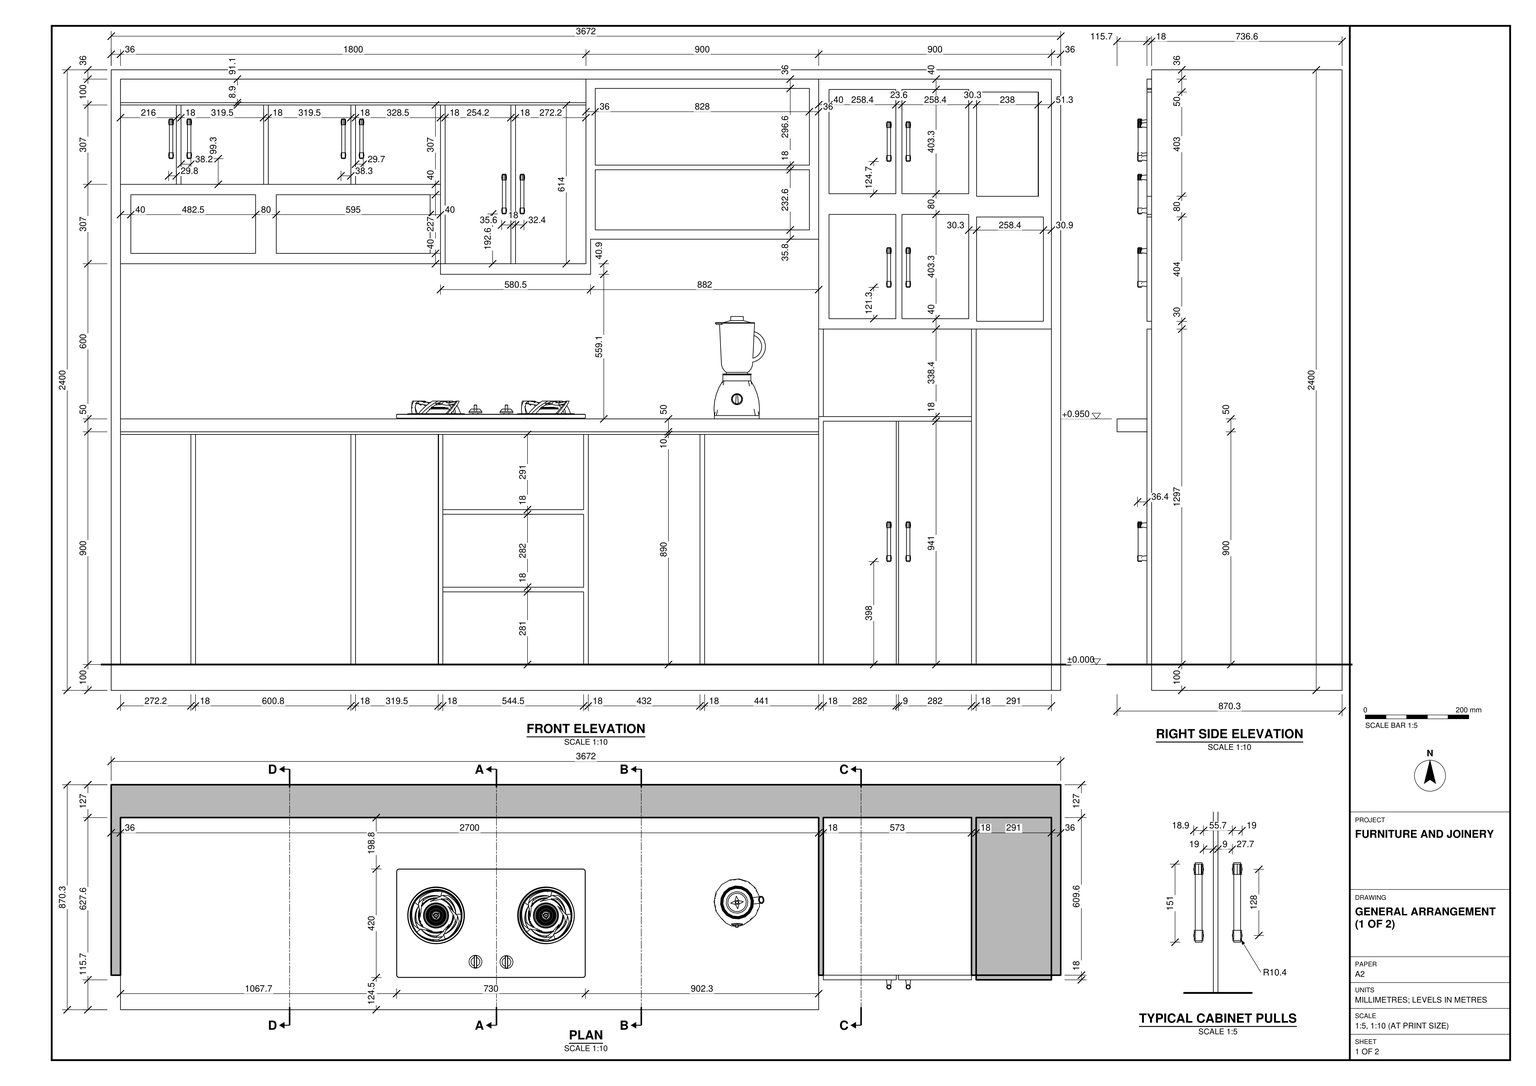
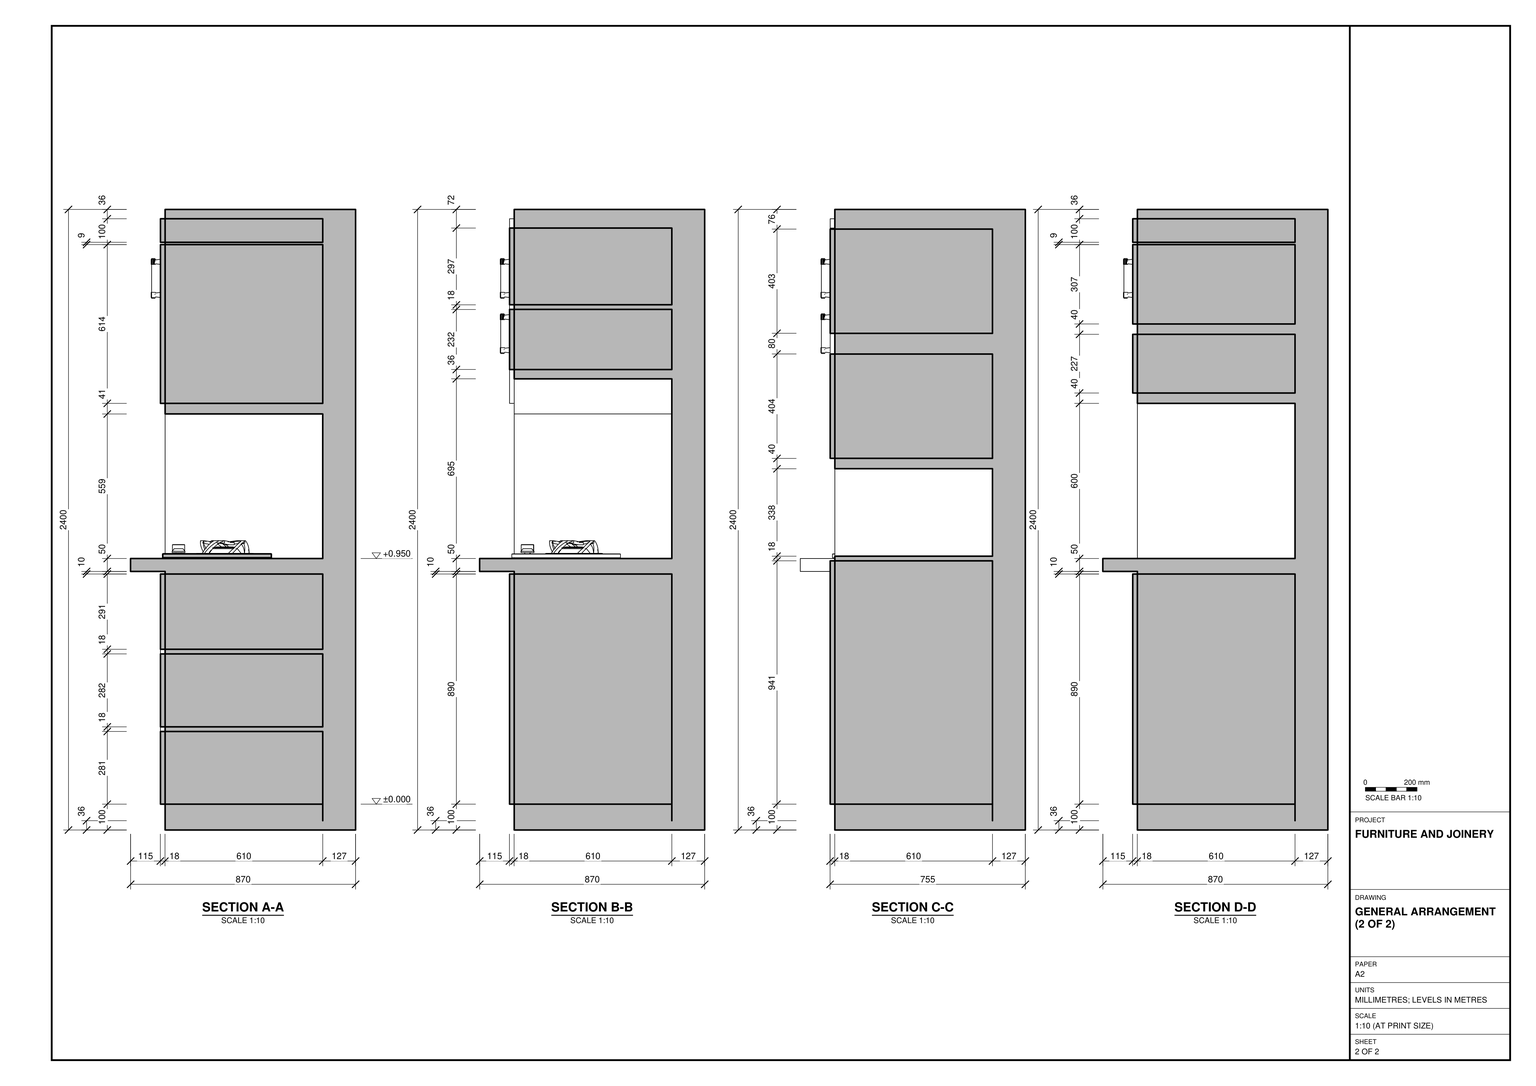
Build the fitted kitchen joinery in SketchUp from task_files/diagram_01.pdf. Work in millimetres. The complete unit is 3672 mm wide, 870.3 mm deep and 2400 mm high. Use the floor line marked ±0.000 as the 0 mm datum. The base of the surround is 100 mm below this line, and the worktop surface is 950 mm above it.

Use the plan and front elevation to lay out the backing, end panels, base cabinets and upper cabinets. Run the worktop across the left-hand base cabinets and stop it at the tall storage section on the right. Use the sections on the second sheet to set the panel thicknesses, shelf heights and projection of the worktop beyond the cabinet fronts. Match the stacked compartments below the cooktop, the changing heights of the upper cupboards and the open shelf bay beside them. Fit vertical pulls to the doors indicated in the elevation. Place the cooktop and countertop mixer in their plan positions.

Make the surround, worktop and each distinct cabinet assembly separate groups or components, and use components for repeated parts such as pulls. Appliances, decor and loose items may be any suitable library components. Save one SketchUp model as output_files/fitted_kitchen_cabinet_run_with_a_projecting_worktop.skp.

# SketchUp Ruby script. Lengths in millimetres.
U = 1.mm
M = Sketchup.active_model
def pt(a) = Geom::Point3d.new(a.map { |v| v * U })
def face(e, loops, mat)
  f = e.add_face(loops[0].map { |a| pt(a) })
  loops[1..].each { |l| e.add_face(l.map { |a| pt(a) }).erase! }
  f.material = f.back_material = mat if mat
  f
end
# faces: each face lists its corners as indices into pts; further lists are holes
def faces(e, pts, list, mat = nil) = list.each { |f| face(e, (f[0].is_a?(Array) ? f : [f]).map { |l| l.map { |i| pts[i] } }, mat) }
# xy, xz, yz: faces in a plane at the given z, y or x. An outline is a flat list of corners, or four numbers for a rectangle; further outlines are holes
def ring(l) = l.size == 4 ? [[l[0], l[1]], [l[2], l[1]], [l[2], l[3]], [l[0], l[3]]] : l.each_slice(2).to_a
def flat(e, list, mat, &to3) = list.each { |f| face(e, (f[0].is_a?(Array) ? f : [f]).map { |l| ring(l).map { |u, v| to3.(u, v) } }, mat) }
def xy(e, z, list, mat = nil) = flat(e, list, mat) { |x, y| [x, y, z] }
def xz(e, y, list, mat = nil) = flat(e, list, mat) { |x, z| [x, y, z] }
def yz(e, x, list, mat = nil) = flat(e, list, mat) { |y, z| [x, y, z] }
def lines(e, pts, list) = list.each { |a, b| e.add_line(pt(pts[a]), pt(pts[b])) }
# prism: a flat outline (further loops are holes) pulled along v
def prism(e, loops, v, mat = nil)
  f = face(e, loops, mat); d = Geom::Vector3d.new(v.map { |x| x * U })
  f.pushpull(f.normal.samedirection?(d) ? d.length : -d.length)
end
def box(e, o, s, mat = nil) = prism(e, [[o, [o[0] + s[0], o[1], o[2]], [o[0] + s[0], o[1] + s[1], o[2]], [o[0], o[1] + s[1], o[2]]]], [0, 0, s[2]], mat)
def at(x, y, z, deg = 0) = Geom::Transformation.translation(pt([x, y, z])) * Geom::Transformation.rotation(ORIGIN, Z_AXIS, deg.degrees)
def axes(o, x, y, z) = Geom::Transformation.new([*x, 0, *y, 0, *z, 0, *pt(o).to_a, 1])
def part(name) = M.definitions.add(name)
# library, detail: a bought-in or finely detailed component or shape, given as its bounding box
def library(name, o, s) = part(name).tap { |d| box(d.entities, o, s) }
def detail(e, o, s) = box(e.add_group.entities, o, s)
def put(e, d, t, mat = nil) = e.add_instance(d, t).tap { |i| i.material = mat if mat }
def group(e, t, mat = nil) = e.add_group.tap { |g| g.transformation = t; g.material = mat if mat }.entities
root = M.entities
M.materials.add("0257 AP 9616 Wisteria Lane-N").color = [173, 152, 201]
M.materials.add("0466 AP 9679 Little Andaman-N").color = [89, 168, 184]
M.materials.add("0522 AP 7474 SAPPHIRE ICE").color = [176, 207, 204]
M.materials.add("CLC2-PC-Blanc INTER").color = [249, 249, 249]
M.materials.add("[Color M00]").color = [255, 255, 255]
M.materials.add("[Color M09]").color = [0, 0, 0]
M.materials.add("[Translucent Glass Blue]").color = [100, 149, 237]
M.materials["[Translucent Glass Blue]"].alpha = 0.5
M.materials.add("[Wood Floor]").color = [155, 105, 61]
c1 = library("2-PRODUITS CUISINE CLC2",[-33.7,-33.7,0],[67.4,67.4,274.4])
c2 = library("1-PRODUITS CUISINE CLC2\#1",[-28.3,-28.3,0],[56.6,56.6,273])
c3 = library("GasStove_Black",[0,0,0],[730,420,69])
c4 = part("CLC2-Ele02")
prism(c4.entities,[[[-0.2,-8.1,4],[-0.2,-8.3,0.4],[-0.2,-8.7,-3.2],[-0.2,-9.2,-6.8],[-0.2,-9.9,-10.3],[-0.2,-10.8,-13.9],[-0.2,-11.8,-17.3],[-0.2,-13,-20.8],[-0.2,-5.2,-21.4],[-0.2,-1.7,21.4],[-0.2,-9.5,22.1],[-0.2,-8.9,18.5],[-0.2,-8.5,14.9],[-0.2,-8.2,11.3],[-0.2,-8.1,7.7]]],[-21.2,0,0],"[Color M00]")
xy(c4.entities,-40,[[-36.6,-4.9,36.6,0]],"CLC2-PC-Blanc INTER")
xy(c4.entities,-38,[[-34.9,-2.9,34.9,0]],"CLC2-PC-Blanc INTER")
xy(c4.entities,-22,[[-21.5,-7.3,21.5,-2.9]],"CLC2-PC-Blanc INTER")
xy(c4.entities,22,[[-21.5,-7.3,21.5,-2.9]],"CLC2-PC-Blanc INTER")
xy(c4.entities,38,[[-34.9,-2.9,34.9,0]],"CLC2-PC-Blanc INTER")
xy(c4.entities,40,[[-36.6,-4.9,36.6,0]],"CLC2-PC-Blanc INTER")
xz(c4.entities,-8.1,[[0.2,4,21.4,7.7]],"[Color M00]")
xz(c4.entities,-2.9,[[[-34.9,-38,-35.7,-33.1,-36.5,-26.5,-37.2,-19.9,-37.7,-13.3,-38,-6.6,-38,6.6,-37.7,13.3,-37.2,19.9,-36.5,26.5,-35.7,33.1,-34.9,38,34.9,38,35.7,33.1,36.5,26.5,37.2,19.9,37.7,13.3,38,6.6,38,-6.6,37.7,-13.3,37.2,-19.9,36.5,-26.5,35.7,-33.1,34.9,-38],[-21.5,-22,21.5,22]]],"CLC2-PC-Blanc INTER")
xz(c4.entities,0,[[-36.6,-40,-37.6,-33.4,-38.5,-26.7,-39.1,-20.1,-39.6,-13.4,-39.9,-6.7,-40,0,-39.9,6.7,-39.6,13.4,-39.1,20.1,-38.5,26.7,-37.6,33.4,-36.6,40,0,40,0,38,-34.9,38,-35.7,33.1,-36.5,26.5,-37.2,19.9,-37.7,13.3,-38,6.6,-38,-6.6,-37.7,-13.3,-37.2,-19.9,-36.5,-26.5,-35.7,-33.1,-34.9,-38,0,-38,0,-40],[0,-40,0,-38,34.9,-38,35.7,-33.1,36.5,-26.5,37.2,-19.9,37.7,-13.3,38,-6.6,38,6.6,37.7,13.3,37.2,19.9,36.5,26.5,35.7,33.1,34.9,38,0,38,0,40,36.6,40,37.6,33.4,38.5,26.7,39.1,20.1,39.6,13.4,39.9,6.7,40,0,39.9,-6.7,39.6,-13.4,39.1,-20.1,38.5,-26.7,37.6,-33.4,36.6,-40]],"CLC2-PC-Blanc INTER")
yz(c4.entities,-38,[[-2.9,-6.6,0,0],[-2.9,0,0,6.6]],"CLC2-PC-Blanc INTER")
yz(c4.entities,-21.5,[[-7.3,-22,-2.9,-22,-2.9,22,-7.3,22,-7.5,20.1,-8,13.4,-8.2,6.7,-8.3,0,-8.2,-6.7,-8,-13.4,-7.5,-20.1]],"CLC2-PC-Blanc INTER")
yz(c4.entities,0.2,[[-5.2,-21.4,-13,-20.8,-11.8,-17.3,-10.8,-13.9,-9.9,-10.3,-9.2,-6.8,-8.7,-3.2,-8.3,0.4,-8.1,4,-8.1,7.7,-8.2,11.3,-8.5,14.9,-8.9,18.5,-9.5,22.1,-1.7,21.4]],"[Color M09]")
yz(c4.entities,21.4,[[-5.2,-21.4,-1.7,21.4,-9.5,22.1,-8.9,18.5,-8.5,14.9,-8.2,11.3,-8.1,7.7,-8.1,4,-8.3,0.4,-8.7,-3.2,-9.2,-6.8,-9.9,-10.3,-10.8,-13.9,-11.8,-17.3,-13,-20.8]],"[Color M09]")
yz(c4.entities,21.5,[[-7.3,-22,-7.5,-20.1,-8,-13.4,-8.2,-6.7,-8.3,0,-8.2,6.7,-8,13.4,-7.5,20.1,-7.3,22,-2.9,22,-2.9,-22]],"CLC2-PC-Blanc INTER")
yz(c4.entities,38,[[-2.9,-6.6,0,0],[-2.9,0,0,6.6]],"CLC2-PC-Blanc INTER")
p = [[-33.5,-8,13.4],[-34,-7.5,20.1],[-34.7,-6.8,26.7],[-35.5,-6,33.4],[-36.6,-4.9,40],[-37.6,-3.9,33.4],
  [-38.5,-3,26.7],[-39.1,-2.4,20.1],[-39.6,-1.9,13.4],[-39.9,-1.6,6.7],[-40,-1.5,0],[-39.9,-1.6,-6.7],
  [-39.6,-1.9,-13.4],[-39.1,-2.4,-20.1],[-38.5,-3,-26.7],[-37.6,-3.9,-33.4],[-36.6,-4.9,-40],[-35.5,-6,-33.4],
  [-34.7,-6.8,-26.7],[-34,-7.5,-20.1],[-33.5,-8,-13.4],[-33.2,-8.2,-6.7],[-33.1,-8.3,0],[-33.2,-8.2,6.7],
  [34,-7.5,20.1],[33.5,-8,13.4],[33.2,-8.2,6.7],[33.1,-8.3,0],[33.2,-8.2,-6.7],[33.5,-8,-13.4],
  [34,-7.5,-20.1],[34.7,-6.8,-26.7],[35.5,-6,-33.4],[36.6,-4.9,-40],[37.6,-3.9,-33.4],[38.5,-3,-26.7],
  [39.1,-2.4,-20.1],[39.6,-1.9,-13.4],[39.9,-1.6,-6.7],[40,-1.5,0],[39.9,-1.6,6.7],[39.6,-1.9,13.4],
  [39.1,-2.4,20.1],[38.5,-3,26.7],[37.6,-3.9,33.4],[36.6,-4.9,40],[35.5,-6,33.4],[34.7,-6.8,26.7],
  [-36.6,0,-40],[-37.6,0,-33.4],[36.6,0,-40],[37.6,0,-33.4],[-34.9,0,-38],[-35.7,0,-33.1],
  [-35.7,-2.9,-33.1],[-34.9,-2.9,-38],[35.7,0,-33.1],[34.9,0,-38],[34.9,-2.9,-38],[35.7,-2.9,-33.1],
  [-38.5,0,-26.7],[38.5,0,-26.7],[-36.5,0,-26.5],[-36.5,-2.9,-26.5],[36.5,0,-26.5],[36.5,-2.9,-26.5],
  [21.5,-7.3,-22],[-21.5,-7.3,-22],[-21.5,-7.5,-20.1],[-33.7,-7.5,-20.1],[33.7,-7.5,-20.1],[21.5,-7.5,-20.1],
  [-39.1,0,-20.1],[39.1,0,-20.1],[-37.2,0,-19.9],[-37.2,-2.9,-19.9],[37.2,0,-19.9],[37.2,-2.9,-19.9],
  [0.2,-13,-20.8],[0.2,-5.2,-21.4],[21.4,-5.2,-21.4],[21.4,-13,-20.8],[0.2,-1.7,21.4],[21.4,-1.7,21.4],
  [0.2,-11.8,-17.3],[21.4,-11.8,-17.3],[-21.5,-8,-13.4],[21.5,-8,-13.4],[-39.6,0,-13.4],[39.6,0,-13.4],
  [-37.7,0,-13.3],[-37.7,-2.9,-13.3],[37.7,0,-13.3],[37.7,-2.9,-13.3],[0.2,-10.8,-13.9],[21.4,-10.8,-13.9],
  [0.2,-9.9,-10.3],[21.4,-9.9,-10.3],[-21.5,-8.2,-6.7],[21.5,-8.2,-6.7],[-39.9,0,-6.7],[39.9,0,-6.7],
  [-38,0,-6.6],[-38,-2.9,-6.6],[38,0,-6.6],[38,-2.9,-6.6],[0.2,-9.2,-6.8],[21.4,-9.2,-6.8],
  [0.2,-8.7,-3.2],[21.4,-8.7,-3.2],[-21.5,-8.3,0],[21.5,-8.3,0],[-40,0,0],[40,0,0],
  [0.2,-8.3,0.4],[21.4,-8.3,0.4],[-21.5,-8.2,6.7],[21.5,-8.2,6.7],[-39.9,0,6.7],[39.9,0,6.7],
  [0.2,-8.1,4],[21.4,-8.1,4],[-38,0,6.6],[-37.7,0,13.3],[-37.7,-2.9,13.3],[-38,-2.9,6.6],
  [37.7,0,13.3],[38,0,6.6],[38,-2.9,6.6],[37.7,-2.9,13.3],[-21.5,-8,13.4],[21.5,-8,13.4],
  [-39.6,0,13.4],[39.6,0,13.4],[0.2,-8.2,11.3],[0.2,-8.1,7.7],[21.4,-8.1,7.7],[21.4,-8.2,11.3],
  [0.2,-8.5,14.9],[21.4,-8.5,14.9],[-37.2,0,19.9],[-37.2,-2.9,19.9],[37.2,0,19.9],[37.2,-2.9,19.9],
  [-21.5,-7.5,20.1],[-33.7,-7.5,20.1],[33.7,-7.5,20.1],[21.5,-7.5,20.1],[-39.1,0,20.1],[39.1,0,20.1],
  [0.2,-8.9,18.5],[21.4,-8.9,18.5],[0.2,-9.5,22.1],[21.4,-9.5,22.1],[-36.5,0,26.5],[-36.5,-2.9,26.5],
  [36.5,0,26.5],[36.5,-2.9,26.5],[-21.5,-7.3,22],[21.5,-7.3,22],[-38.5,0,26.7],[38.5,0,26.7],
  [-35.7,0,33.1],[-35.7,-2.9,33.1],[35.7,0,33.1],[35.7,-2.9,33.1],[-37.6,0,33.4],[37.6,0,33.4],
  [-34.9,0,38],[-34.9,-2.9,38],[34.9,0,38],[34.9,-2.9,38],[-36.6,0,40],[36.6,0,40]]
faces(c4.entities,p,[[0,1,2,3,4,5,6,7,8,9,10,11,12,13,14,15,16,17,18,19,20,21,22,23],[24,25,26,27,28,29,30,31,32,33,34,35,36,37,38,39,40,41,42,43,44,45,46,47],[32,17,16,33],[31,18,17,32],[66,67,68,69,19,18,31,30,70,71],[78,79,80,81],[79,82,83,80],[69,68,86,20,19],
  [71,70,30,29,87],[20,86,98,21],[87,29,28,99],[21,98,110,22],[99,28,27,111],[22,110,116,23],[111,27,26,117],[23,116,130,0],
  [117,26,25,131],[0,130,144,145,1],[131,25,24,146,147],[144,158,159,147,146,24,47,2,1,145],[82,152,153,83],[46,3,2,47],[4,3,46,45]],"[Color M09]")
faces(c4.entities,p,[[48,16,15,49],[33,50,51,34],[52,53,54,55],[56,57,58,59],[49,15,14,60],[34,51,61,35],[53,62,63,54],[64,56,59,65],
  [60,14,13,72],[35,61,73,36],[62,74,75,63],[76,64,65,77],[72,13,12,88],[36,73,89,37],[74,90,91,75],[92,76,77,93],
  [88,12,11,100],[37,89,101,38],[90,102,103,91],[104,92,93,105],[100,11,10,112],[38,101,113,39],[112,10,9,118],[39,113,119,40],
  [122,123,124,125],[126,127,128,129],[118,9,8,132],[40,119,133,41],[123,140,141,124],[142,126,129,143],[132,8,7,148],[41,133,149,42],
  [140,154,155,141],[156,142,143,157],[148,7,6,160],[42,149,161,43],[154,162,163,155],[164,156,157,165],[160,6,5,166],[43,161,167,44],
  [162,168,169,163],[170,164,165,171],[166,5,4,172],[44,167,173,45]],"CLC2-PC-Blanc INTER")
faces(c4.entities,p,[[84,78,81,85],[94,84,85,95],[96,94,95,97],[106,96,97,107],[108,106,107,109],[114,108,109,115],[120,114,115,121],[134,135,136,137],
  [138,134,137,139],[150,138,139,151],[152,150,151,153]],"[Color M00]")
c5 = part("2-PRISEELC CLC2")
put(c5.entities,c4,axes([0,0,0],[1,0,0],[0,0,-1],[0,1,0]),"[Color M09]")
c6 = library("mixer",[64.3,72.1,0],[208.3,190.8,396])
c7 = library("1-POIGNEE CLC2",[-77,-9.5,0],[154,19,36])
c8 = part("Group\#3")
prism(c8.entities,[[[258.4,-18,0],[0,-18,0],[0,0,0],[238,0,0],[239.3,0,0],[258.4,0,0]]],[0,0,403.3])
c9 = part("Group\#9")
box(c9.entities,[0,-18,0],[254.3,18,614])
c10 = part("Group\#10")
box(c10.entities,[0,-18,0],[482.5,18,227])
c11 = part("Group\#15")
box(c11.entities,[0,-18,0],[282,18,941])
c12 = part("Group\#22")
box(c12.entities,[0,-18,0],[432,18,890])
put(root,c1,at(2088.8,471.5,2031.4))
put(root,c2,axes([1996.6,349.6,1780.8],[1,0,0],[0,1,0],[0,0,0.67]))
put(root,c3,at(1103.7,124.5,1050))
put(root,c5,axes([2150.3,743.3,1460.7],[1,0,0],[0,0,1],[0,-1,0]),"[Color M09]")
put(root,c6,at(2264.9,243.1,1050))
put(root,c7,axes([231.6,115.7,2133.3],[0,0,-1],[1,0,0],[0,-1,0]))
put(root,c7,axes([301.6,115.7,2133.3],[0,0,-1],[1,0,0],[0,-1,0]))
put(root,c7,axes([968.1,115.7,2133.3],[0,0,-1],[1,0,0],[0,-1,0]))
put(root,c7,axes([898.1,115.7,2133.3],[0,0,-1],[1,0,0],[0,-1,0]))
put(root,c7,axes([1589.6,115.7,1919.6],[0,0,-1],[1,0,0],[0,-1,0]))
put(root,c7,axes([1519.6,115.7,1919.6],[0,0,-1],[1,0,0],[0,-1,0]))
put(root,c7,axes([3007.6,115.7,2122.4],[0,0,-1],[1,0,0],[0,-1,0]))
put(root,c7,axes([3082.2,115.7,2122.4],[0,0,-1],[1,0,0],[0,-1,0]))
put(root,c7,axes([3082.2,115.7,1635.7],[0,0,-1],[1,0,0],[0,-1,0]))
put(root,c7,axes([3007.6,115.7,1635.7],[0,0,-1],[1,0,0],[0,-1,0]))
put(root,c7,axes([3082.2,115.7,575],[0,0,-1],[1,0,0],[0,-1,0]))
put(root,c7,axes([3007.6,115.7,575],[0,0,-1],[1,0,0],[0,-1,0]))
g1 = group(root,at(3058,133.7,1920.7),"[Translucent Glass Blue]")
prism(g1,[[[238,0,0],[239.3,0,0],[258.4,0,0],[258.4,-18,0],[0,-18,0],[0,0,0]]],[0,0,403.3])
g2 = group(root,at(3346.7,133.7,1910.7),"[Translucent Glass Blue]")
xy(g2,0,[[0,-18,238,0],[238,-18,239.3,0]])
xy(g2,403.3,[[0,-18,239.3,0]])
xz(g2,-18,[[0,0,239.3,403.3]])
xz(g2,0,[[0,0,238,403.3],[238,0,239.3,403.3]])
yz(g2,0,[[-18,0,0,403.3]])
yz(g2,239.3,[[-18,0,0,403.3]])
put(root,c8,at(2776,133.7,1920.7),"[Translucent Glass Blue]")
put(root,c8,at(2776,133.7,1437.4),"[Translucent Glass Blue]")
put(root,c8,at(3058,133.7,1437.4),"[Translucent Glass Blue]")
put(root,c8,at(3346.7,133.7,1427.4),"0466 AP 9679 Little Andaman-N")
g3 = group(root,at(36,133.7,2272.9),"0466 AP 9679 Little Andaman-N")
box(g3,[0,-18,0],[1800,18,91.1])
g4 = group(root,at(36,133.7,1957),"0257 AP 9616 Wisteria Lane-N")
box(g4,[0,-18,0],[216,18,307])
g5 = group(root,at(270,133.7,1957),"0257 AP 9616 Wisteria Lane-N")
box(g5,[0,-18,0],[319.5,18,307])
g6 = group(root,at(607.5,133.7,1957),"0257 AP 9616 Wisteria Lane-N")
box(g6,[0,-18,0],[319.5,18,307])
g7 = group(root,at(945,133.7,1957),"0257 AP 9616 Wisteria Lane-N")
box(g7,[0,-18,0],[328.5,18,307])
put(root,c9,at(1291.5,133.7,1650),"0466 AP 9679 Little Andaman-N")
put(root,c9,axes([1563.7,133.7,1650],[1.0708,0,0],[0,1,0],[0,0,1]),"0466 AP 9679 Little Andaman-N")
put(root,c10,at(76,133.7,1690),"[Translucent Glass Blue]")
put(root,c10,axes([638.5,133.7,1690],[1.23316,0,0],[0,1,0],[0,0,1]),"[Translucent Glass Blue]")
g8 = group(root,at(1872,133.7,1780.8),"[Translucent Glass Blue]")
box(g8,[0,-18,0],[828,18,232.6])
g9 = group(root,at(1872,133.7,2031.4),"[Translucent Glass Blue]")
box(g9,[0,-18,0],[828,18,296.6])
g10 = group(root,at(3345,133.7,100),"0257 AP 9616 Wisteria Lane-N")
box(g10,[0,-18,0],[291,18,1297.4])
put(root,c11,at(3045,133.7,100),"0522 AP 7474 SAPPHIRE ICE")
put(root,c11,at(2754,133.7,100),"0522 AP 7474 SAPPHIRE ICE")
g11 = group(root,at(0,743.3,0),"[Wood Floor]")
xy(g11,0,[[0,-609.6,3672,127]])
xy(g11,100,[[36,-609.6,308.3,0],[308.3,-609.6,317.3,0],[317.3,-609.6,326.3,0],[326.3,-609.6,927,0],[927,-609.6,936,0],
  [936,-609.6,945,0],[945,-609.6,1264.5,0],[1264.5,-609.6,1273.5,0],[1273.5,-609.6,1282.5,0],[1282.5,-609.6,1554.8,0],
  [1554.8,-609.6,1827,0],[1827,-609.6,1836,0],[1836,-609.6,1845,0],[1845,-609.6,2277,0],[2277,-609.6,2286,0],
  [2286,-609.6,2295,0],[2295,-609.6,2736,0],[2736,-609.6,2754,0],[2754,-609.6,3027,0],[3027,-609.6,3036,0],
  [3036,-609.6,3045,0],[3045,-609.6,3327,0],[3327,-609.6,3336,0],[3336,-609.6,3345,0],[3345,-609.6,3636,0]])
xy(g11,381,[[1282.5,-609.6,1554.8,0],[1554.8,-609.6,1827,0]])
xy(g11,399,[[1282.5,-609.6,1554.8,0],[1554.8,-609.6,1827,0]])
xy(g11,681,[[1282.5,-609.6,1554.8,0],[1554.8,-609.6,1827,0]])
xy(g11,699,[[1282.5,-609.6,1554.8,0],[1554.8,-609.6,1827,0]])
xy(g11,990,[[36,-609.6,308.3,0],[326.3,-609.6,927,0],[945,-609.6,1264.5,0],[1282.5,-609.6,1827,0],[1845,-609.6,2277,0],
  [2277,-609.6,2286,0],[2286,-609.6,2295,0],[2295,-609.6,2736,0]])
xy(g11,1000,[[36,-743.3,936,-609.6],[936,-743.3,1273.5,-609.6],[1273.5,-743.3,1554.8,-609.6],[1554.8,-743.3,1836,-609.6],[1836,-743.3,2736,-609.6]])
xy(g11,1041,[[2754,-609.6,3027,0],[3045,-609.6,3327,0]])
xy(g11,1050,[[36,-743.3,2736,0]])
xy(g11,1059,[[2754,-609.6,3327,0]])
xy(g11,1397.4,[[2754,-609.6,3327,0],[3345,-609.6,3636,0]])
xy(g11,1437.4,[[2776,-609.6,3014,0],[3058,-609.6,3316.4,0]])
xy(g11,1447.4,[[3346.7,-609.6,3586,0]])
xy(g11,1609.1,[[1273.5,-609.6,1854,0]])
xy(g11,1650,[[36,-609.6,1273.5,0],[1291.5,-609.6,1545.8,0],[1563.8,-609.6,1836,0]])
xy(g11,1690,[[76,-609.6,558.5,0],[638.5,-609.6,1233.5,0]])
xy(g11,1744.8,[[1854,-609.6,2736,0]])
xy(g11,1780.8,[[1872,-609.6,2700,0]])
xy(g11,1830.7,[[3346.7,-609.6,3586,0]])
xy(g11,1840.7,[[2776,-609.6,3014,0],[3058,-609.6,3316.4,0]])
xy(g11,1917,[[76,-609.6,558.5,0],[638.5,-609.6,1233.5,0]])
xy(g11,1920.7,[[2776,-609.6,3014,0],[3058,-609.6,3316.4,0]])
xy(g11,1930.7,[[3346.7,-609.6,3586,0]])
xy(g11,1957,[[36,-609.6,252,0],[270,-609.6,589.5,0],[607.5,-609.6,927,0],[945,-609.6,1273.5,0]])
xy(g11,2013.4,[[1872,-609.6,2700,0]])
xy(g11,2031.4,[[1872,-609.6,2700,0]])
xy(g11,2264,[[36,-609.6,252,0],[270,-609.6,589.5,0],[607.5,-609.6,927,0],[945,-609.6,1273.5,0],[1291.5,-609.6,1545.8,0],
  [1563.8,-609.6,1836,0]])
xy(g11,2272.9,[[36,-609.6,37.3,0],[37.3,-609.6,937.3,0],[937.3,-609.6,1836,0]])
xy(g11,2314,[[3346.7,-609.6,3586,0]])
xy(g11,2324,[[2776,-609.6,3014,0],[3058,-609.6,3316.4,0]])
xy(g11,2328,[[1872,-609.6,2700,0]])
xy(g11,2364,[[36,-609.6,1836,0]])
xy(g11,2400,[[0,-609.6,3672,127]])
xz(g11,-743.3,[[36,1000,2736,1050]])
xz(g11,-609.6,[[0,0,1273.5,0,1273.5,100,36,100,36,2364,3636,2364,3636,0,3672,0,3672,2400,0,2400],[1273.5,0,1554.8,100],[1554.8,0,1836,100],[1836,0,2736,100],[2736,0,3036,100],
  [3036,0,3336,100],[3336,0,3636,100],[308.3,100,326.3,990],[927,100,945,990],[1264.5,100,1282.5,990],
  [1827,100,1845,100,1845,990,1827,990,1827,699,1282.5,699,1282.5,681,1827,681,1827,399,1282.5,399,1282.5,381,1827,381],[2277,100,2295,990],[2736,100,2754,100,2754,1041,3327,1041,3327,1059,2736,1059],[3027,100,3045,1041],[3327,100,3345,1397.4],
  [36,990,2736,1000],[2736,1059,2754,1397.4],[[2736,1397.4,3636,2364],[3058,1920.7,3316.4,2324],[3058,1437.4,3316.4,1840.7],[2776,1437.4,3014,1840.7],[2776,1920.7,3014,2324],[3346.7,1930.7,3586,2314],[3346.7,1447.4,3586,1830.7]],[[1273.5,1609.1,1854,1609.1,1854,1744.8,2736,1744.8,2736,2364,1836,2364,1836,1650,1273.5,1650],[1872,2031.4,2700,2328],[1872,1780.8,2700,2013.4]],[[36,1650,1273.5,1957],[638.5,1690,1233.5,1917],[76,1690,558.5,1917]],
  [1273.5,1650,1291.5,2264],[1545.8,1650,1563.8,2264],[252,1957,270,2264],[589.5,1957,607.5,2264],[927,1957,945,2264],
  [36,2264,1836,2272.9]])
xz(g11,0,[[36,36,1273.5,100],[1273.5,36,1554.8,100],[1554.8,36,1836,100],[1836,36,2736,100],[2736,36,3036,100],
  [3036,36,3336,100],[3336,36,3636,75.9],[3336,75.9,3636,100],[36,100,308.3,990],[326.3,100,927,990],
  [945,100,1264.5,990],[1282.5,100,1827,381],[1845,100,2277,990],[2295,100,2736,990],[2754,100,3027,1041],
  [3045,100,3327,1041],[3345,100,3636,1397.4],[1282.5,399,1827,681],[1282.5,699,1827,990],[36,1050,2736,1050,2736,1744.8,1854,1744.8,1854,1609.1,1273.5,1609.1,1273.5,1650,36,1650],
  [2754,1059,3327,1397.4],[2776,1437.4,3014,1840.7],[3058,1437.4,3316.4,1840.7],[3346.7,1447.4,3586,1830.7],[1291.5,1650,1545.8,2264],
  [1563.8,1650,1836,2264],[76,1690,558.5,1917],[638.5,1690,1233.5,1917],[1872,1780.8,2700,2013.4],[2776,1920.7,3014,2324],
  [3058,1920.7,3316.4,2324],[3346.7,1930.7,3586,2314],[36,1957,252,2264],[270,1957,589.5,2264],[607.5,1957,927,2264],
  [945,1957,1273.5,2264],[1872,2031.4,2700,2328],[36,2272.9,1836,2364]])
xz(g11,127,[[0,0,3672,2400]])
yz(g11,0,[[-609.6,0,127,2400]])
yz(g11,36,[[-609.6,100,0,990],[-743.3,1000,-609.6,1050],[-609.6,1050,0,1650],[-609.6,1957,0,2264],[-609.6,2272.9,0,2364]])
yz(g11,76,[[-609.6,1690,0,1917]])
yz(g11,252,[[-609.6,1957,0,2264]])
yz(g11,270,[[-609.6,1957,0,2264]])
yz(g11,308.3,[[-609.6,100,0,990]])
yz(g11,326.3,[[-609.6,100,0,990]])
yz(g11,558.5,[[-609.6,1690,0,1917]])
yz(g11,589.5,[[-609.6,1957,0,2264]])
yz(g11,607.5,[[-609.6,1957,0,2264]])
yz(g11,638.5,[[-609.6,1690,0,1917]])
yz(g11,927,[[-609.6,100,0,990],[-609.6,1957,0,2264]])
yz(g11,945,[[-609.6,100,0,990],[-609.6,1957,0,2264]])
yz(g11,1233.5,[[-609.6,1690,0,1917]])
yz(g11,1264.5,[[-609.6,100,0,990]])
yz(g11,1273.5,[[-609.6,1609.1,0,1650],[-609.6,1957,0,2264]])
yz(g11,1282.5,[[-609.6,100,0,381],[-609.6,399,0,681],[-609.6,699,0,990]])
yz(g11,1291.5,[[-609.6,1650,0,2264]])
yz(g11,1545.8,[[-609.6,1650,0,2264]])
yz(g11,1563.8,[[-609.6,1650,0,2264]])
yz(g11,1827,[[-609.6,100,0,381],[-609.6,399,0,681],[-609.6,699,0,990]])
yz(g11,1836,[[-609.6,1650,0,2264],[-609.6,2272.9,0,2364]])
yz(g11,1845,[[-609.6,100,0,990]])
yz(g11,1854,[[-609.6,1609.1,0,1744.8]])
yz(g11,1872,[[-609.6,1780.8,0,2013.4],[-609.6,2031.4,0,2328]])
yz(g11,2277,[[-609.6,100,0,990]])
yz(g11,2295,[[-609.6,100,0,990]])
yz(g11,2700,[[-609.6,1780.8,0,2013.4],[-609.6,2031.4,0,2328]])
yz(g11,2736,[[-609.6,100,0,990],[-609.6,990,0,1000],[-743.3,1000,-609.6,1050],[-609.6,1050,0,1744.8]])
yz(g11,2754,[[-609.6,100,0,1041],[-609.6,1059,0,1397.4]])
yz(g11,2776,[[-609.6,1437.4,0,1744.8],[-609.6,1744.8,0,1840.7],[-609.6,1920.7,0,2324]])
yz(g11,3014,[[-609.6,1437.4,0,1840.7],[-609.6,1920.7,0,2324]])
yz(g11,3027,[[-609.6,100,0,1041]],"0522 AP 7474 SAPPHIRE ICE")
yz(g11,3045,[[-609.6,100,0,1041]])
yz(g11,3058,[[-609.6,1437.4,0,1840.7],[-609.6,1920.7,0,2324]])
yz(g11,3316.4,[[-609.6,1437.4,0,1840.7],[-609.6,1920.7,0,2324]])
yz(g11,3327,[[-609.6,100,0,1041],[-609.6,1059,0,1397.4]])
yz(g11,3345,[[-609.6,100,0,1397.4]])
yz(g11,3346.7,[[-609.6,1447.4,0,1830.7],[-609.6,1930.7,0,2314]])
yz(g11,3586,[[-609.6,1447.4,0,1830.7],[-609.6,1930.7,0,2314]])
yz(g11,3636,[[-609.6,36,0,100],[-609.6,100,0,1397.4]])
yz(g11,3672,[[-609.6,0,127,2400]])
p = [[1836,0,2272.9],[1837.3,0,2272.9],[1818.7,0,2268.1],[1820,0,2268.1],[36,0,1650],[0,0,1650],
  [261,0,2264],[261,-609.6,2264],[598.5,0,2264],[598.5,-609.6,2264],[936,0,2264],[936,-609.6,2264],
  [1554.8,0,2264],[1554.8,-609.6,2264],[1282.5,0,390],[1282.5,-609.6,390],[1836,0,990],[1836,-606.9,990],
  [1282.5,0,690],[1282.5,-609.6,690],[36,-609.6,36],[36,0,36],[36,0,0],[3636,0,36],
  [3636,0,0],[317.3,0,1000],[317.3,-606.9,1000],[936,0,1000],[936,-606.9,1000],[1273.5,0,1000],
  [1273.5,-606.9,1000],[1554.8,0,1000],[1554.8,-606.9,1000],[1836,0,1000],[1836,-606.9,1000],[1554.8,-609.6,1000],
  [1836,-609.6,1000],[1845,-606.9,381],[1845,-609.6,381],[1845,-606.9,399],[1845,-609.6,399],[1845,-606.9,681],
  [1845,-609.6,681],[1845,-606.9,699],[1845,-609.6,699]]
lines(g11,p,[[0,1],[2,3],[4,5],[6,7],[8,9],[10,11],[12,13],[14,15],[16,17],[18,19],[20,21],[21,22],
  [23,24],[25,26],[27,28],[29,30],[31,32],[33,34],[32,35],[34,36],[37,38],[39,40],[41,42],[43,44]])
g12 = group(g11,at(36,-609.6,100),"0257 AP 9616 Wisteria Lane-N")
prism(g12,[[[272.3,0,890],[272.3,0,0],[0,0,0],[0,0,890],[225,0,890]]],[0,-18,0])
g13 = group(g11,at(326.3,-609.6,100),"0522 AP 7474 SAPPHIRE ICE")
prism(g13,[[[600.8,0,890],[600.8,0,0],[0,0,0],[0,0,890],[225,0,890]]],[0,-18,0])
g14 = group(g11,at(945,-609.6,100),"0522 AP 7474 SAPPHIRE ICE")
prism(g14,[[[321.3,0,890],[321.3,0,0],[0,0,0],[0,0,890],[265.5,0,890]]],[0,-18,0])
g15 = group(g11,at(1282.5,-609.6,699),"0466 AP 9679 Little Andaman-N")
prism(g15,[[[544.5,-18,291],[272.3,-18,291],[0,-18,291],[0,-18,0],[272.3,-18,0],[544.5,-18,0]]],[0,18,0])
g16 = group(g11,at(1282.5,-609.6,399),"0466 AP 9679 Little Andaman-N")
prism(g16,[[[544.5,0,282],[544.5,0,0],[272.3,0,0],[0,0,0],[0,0,282],[272.3,0,282]]],[0,-18,0])
g17 = group(g11,at(1282.5,-609.6,100),"0466 AP 9679 Little Andaman-N")
prism(g17,[[[0,0,0],[0,0,281],[272.3,0,281],[544.5,0,281],[544.5,0,0],[272.3,0,0]]],[0,-18,0])
put(root,c12,at(1845,133.7,100),"0257 AP 9616 Wisteria Lane-N")
put(root,c12,axes([2295,133.7,100],[1.02083,0,0],[0,1,0],[0,0,1]),"0257 AP 9616 Wisteria Lane-N")
